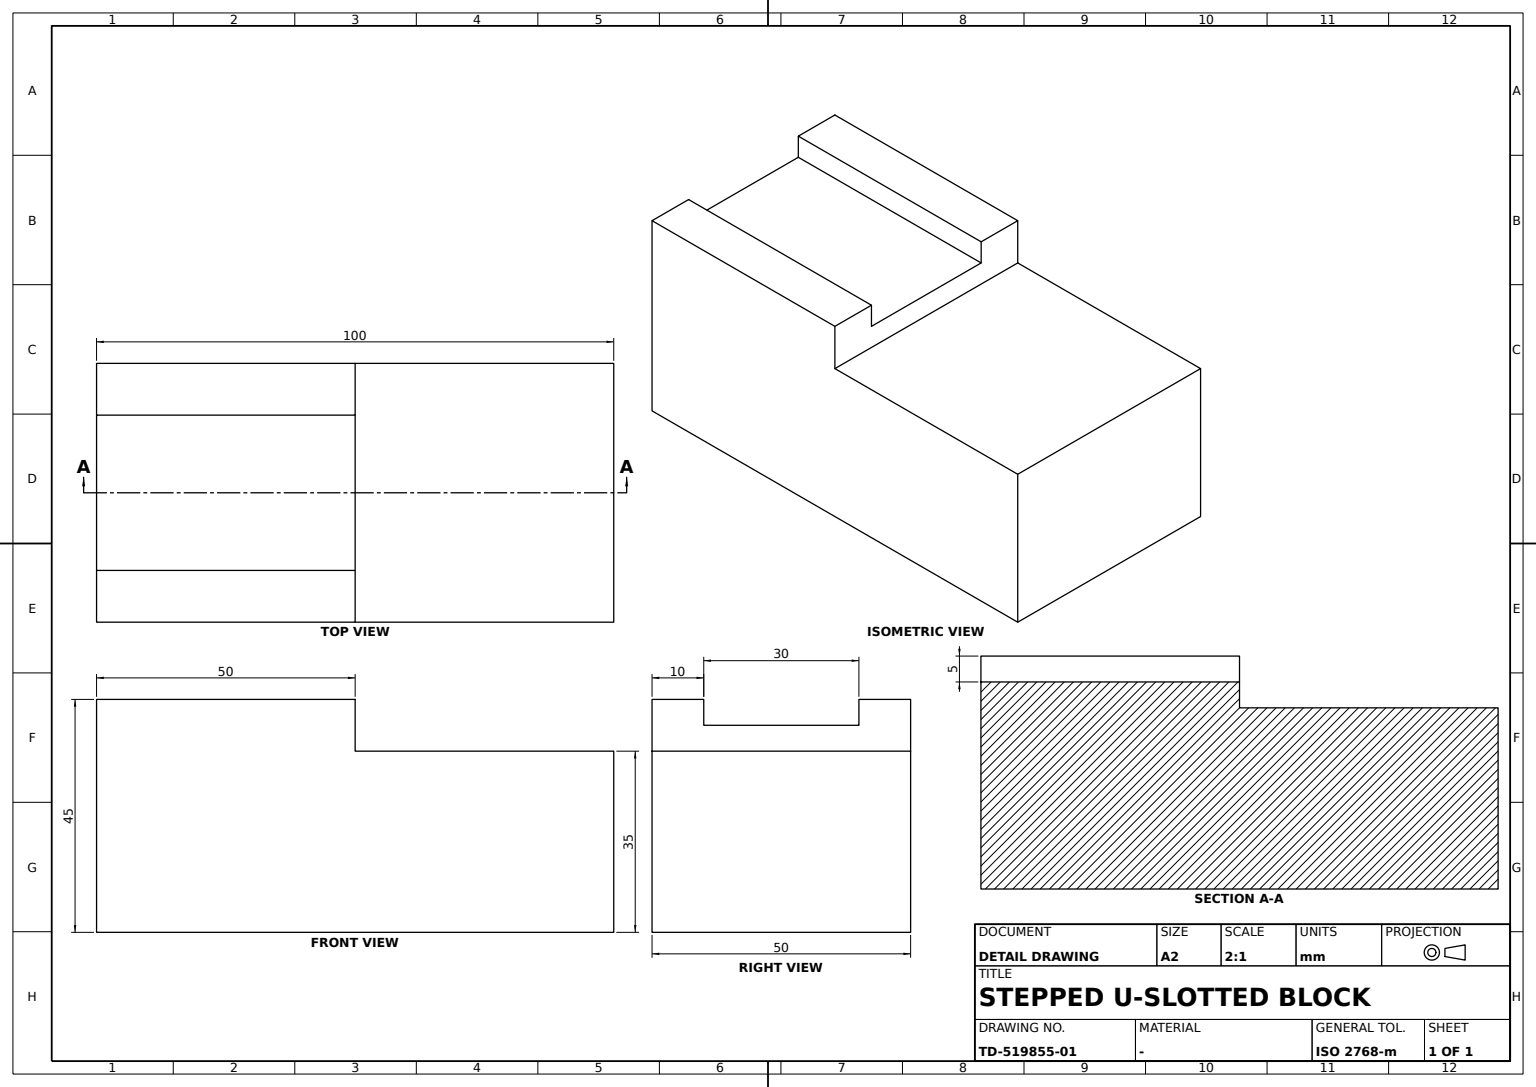
ISO-10303-21;
HEADER;
FILE_DESCRIPTION((''),'2;1');
FILE_NAME('','',(''),(''),'','','');
FILE_SCHEMA(('AUTOMOTIVE_DESIGN'));
ENDSEC;
DATA;
#1=APPLICATION_CONTEXT('');
#2=PRODUCT_CONTEXT('',#1,'mechanical');
#3=PRODUCT('','','',(#2));
#4=PRODUCT_DEFINITION_FORMATION('','',#3);
#5=PRODUCT_DEFINITION_CONTEXT('',#1,'design');
#6=PRODUCT_DEFINITION('','',#4,#5);
#7=PRODUCT_DEFINITION_SHAPE('','',#6);
#8=(LENGTH_UNIT()NAMED_UNIT(*)SI_UNIT(.MILLI.,.METRE.));
#9=(NAMED_UNIT(*)PLANE_ANGLE_UNIT()SI_UNIT($,.RADIAN.));
#10=(NAMED_UNIT(*)SI_UNIT($,.STERADIAN.)SOLID_ANGLE_UNIT());
#11=UNCERTAINTY_MEASURE_WITH_UNIT(LENGTH_MEASURE(1.E-05),#8,'distance_accuracy_value','');
#12=(GEOMETRIC_REPRESENTATION_CONTEXT(3)GLOBAL_UNCERTAINTY_ASSIGNED_CONTEXT((#11))GLOBAL_UNIT_ASSIGNED_CONTEXT((#8,#9,#10))REPRESENTATION_CONTEXT('',''));
#13=CARTESIAN_POINT('',(0.,-40.,5.));
#14=VERTEX_POINT('',#13);
#15=CARTESIAN_POINT('',(-50.,-40.,5.));
#16=VERTEX_POINT('',#15);
#17=CARTESIAN_POINT('',(-25.,-40.,5.));
#18=DIRECTION('',(-1.,0.,0.));
#19=VECTOR('',#18,1000.);
#20=LINE('',#17,#19);
#21=EDGE_CURVE('',#14,#16,#20,.T.);
#22=ORIENTED_EDGE('',*,*,#21,.F.);
#23=CARTESIAN_POINT('',(0.,-10.,5.));
#24=VERTEX_POINT('',#23);
#25=CARTESIAN_POINT('',(0.,-25.,5.));
#26=DIRECTION('',(0.,-1.,0.));
#27=VECTOR('',#26,1000.);
#28=LINE('',#25,#27);
#29=EDGE_CURVE('',#24,#14,#28,.T.);
#30=ORIENTED_EDGE('',*,*,#29,.F.);
#31=CARTESIAN_POINT('',(-50.,-10.,5.));
#32=VERTEX_POINT('',#31);
#33=CARTESIAN_POINT('',(-25.,-10.,5.));
#34=LINE('',#33,#19);
#35=EDGE_CURVE('',#24,#32,#34,.T.);
#36=ORIENTED_EDGE('',*,*,#35,.T.);
#37=CARTESIAN_POINT('',(-50.,-25.,5.));
#38=LINE('',#37,#27);
#39=EDGE_CURVE('',#32,#16,#38,.T.);
#40=ORIENTED_EDGE('',*,*,#39,.T.);
#41=EDGE_LOOP('',(#22,#30,#36,#40));
#42=FACE_OUTER_BOUND('',#41,.T.);
#43=DIRECTION('',(0.,0.,-1.));
#44=AXIS2_PLACEMENT_3D('',#23,#43,#26);
#45=PLANE('',#44);
#46=ADVANCED_FACE('',(#42),#45,.F.);
#47=ORIENTED_EDGE('',*,*,#35,.F.);
#48=CARTESIAN_POINT('',(0.,-10.,10.));
#49=VERTEX_POINT('',#48);
#50=CARTESIAN_POINT('',(0.,-10.,7.5));
#51=VECTOR('',#43,1000.);
#52=LINE('',#50,#51);
#53=EDGE_CURVE('',#49,#24,#52,.T.);
#54=ORIENTED_EDGE('',*,*,#53,.F.);
#55=CARTESIAN_POINT('',(-50.,-10.,10.));
#56=VERTEX_POINT('',#55);
#57=CARTESIAN_POINT('',(-25.,-10.,10.));
#58=LINE('',#57,#19);
#59=EDGE_CURVE('',#49,#56,#58,.T.);
#60=ORIENTED_EDGE('',*,*,#59,.T.);
#61=CARTESIAN_POINT('',(-50.,-10.,7.5));
#62=LINE('',#61,#51);
#63=EDGE_CURVE('',#56,#32,#62,.T.);
#64=ORIENTED_EDGE('',*,*,#63,.T.);
#65=EDGE_LOOP('',(#47,#54,#60,#64));
#66=FACE_OUTER_BOUND('',#65,.T.);
#67=DIRECTION('',(0.,1.,0.));
#68=AXIS2_PLACEMENT_3D('',#48,#67,#43);
#69=PLANE('',#68);
#70=ADVANCED_FACE('',(#66),#69,.F.);
#71=ORIENTED_EDGE('',*,*,#21,.T.);
#72=CARTESIAN_POINT('',(-50.,-40.,10.));
#73=VERTEX_POINT('',#72);
#74=CARTESIAN_POINT('',(-50.,-40.,7.5));
#75=DIRECTION('',(0.,0.,1.));
#76=VECTOR('',#75,1000.);
#77=LINE('',#74,#76);
#78=EDGE_CURVE('',#16,#73,#77,.T.);
#79=ORIENTED_EDGE('',*,*,#78,.T.);
#80=CARTESIAN_POINT('',(0.,-40.,10.));
#81=VERTEX_POINT('',#80);
#82=CARTESIAN_POINT('',(-25.,-40.,10.));
#83=LINE('',#82,#19);
#84=EDGE_CURVE('',#81,#73,#83,.T.);
#85=ORIENTED_EDGE('',*,*,#84,.F.);
#86=CARTESIAN_POINT('',(0.,-40.,7.5));
#87=LINE('',#86,#76);
#88=EDGE_CURVE('',#14,#81,#87,.T.);
#89=ORIENTED_EDGE('',*,*,#88,.F.);
#90=EDGE_LOOP('',(#71,#79,#85,#89));
#91=FACE_OUTER_BOUND('',#90,.T.);
#92=AXIS2_PLACEMENT_3D('',#13,#26,#75);
#93=PLANE('',#92);
#94=ADVANCED_FACE('',(#91),#93,.F.);
#95=CARTESIAN_POINT('',(50.,0.,0.));
#96=VERTEX_POINT('',#95);
#97=CARTESIAN_POINT('',(50.,-50.,0.));
#98=VERTEX_POINT('',#97);
#99=CARTESIAN_POINT('',(50.,-25.,0.));
#100=LINE('',#99,#27);
#101=EDGE_CURVE('',#96,#98,#100,.T.);
#102=ORIENTED_EDGE('',*,*,#101,.T.);
#103=CARTESIAN_POINT('',(50.,-50.,-35.));
#104=VERTEX_POINT('',#103);
#105=CARTESIAN_POINT('',(50.,-50.,-17.5));
#106=LINE('',#105,#51);
#107=EDGE_CURVE('',#98,#104,#106,.T.);
#108=ORIENTED_EDGE('',*,*,#107,.T.);
#109=CARTESIAN_POINT('',(50.,0.,-35.));
#110=VERTEX_POINT('',#109);
#111=CARTESIAN_POINT('',(50.,-25.,-35.));
#112=LINE('',#111,#27);
#113=EDGE_CURVE('',#110,#104,#112,.T.);
#114=ORIENTED_EDGE('',*,*,#113,.F.);
#115=CARTESIAN_POINT('',(50.,0.,-17.5));
#116=LINE('',#115,#51);
#117=EDGE_CURVE('',#96,#110,#116,.T.);
#118=ORIENTED_EDGE('',*,*,#117,.F.);
#119=EDGE_LOOP('',(#102,#108,#114,#118));
#120=FACE_OUTER_BOUND('',#119,.T.);
#121=AXIS2_PLACEMENT_3D('',#95,#18,#43);
#122=PLANE('',#121);
#123=ADVANCED_FACE('',(#120),#122,.F.);
#124=ORIENTED_EDGE('',*,*,#29,.T.);
#125=ORIENTED_EDGE('',*,*,#88,.T.);
#126=CARTESIAN_POINT('',(0.,-50.,10.));
#127=VERTEX_POINT('',#126);
#128=CARTESIAN_POINT('',(0.,-45.,10.));
#129=LINE('',#128,#27);
#130=EDGE_CURVE('',#81,#127,#129,.T.);
#131=ORIENTED_EDGE('',*,*,#130,.T.);
#132=CARTESIAN_POINT('',(0.,-50.,0.));
#133=VERTEX_POINT('',#132);
#134=CARTESIAN_POINT('',(0.,-50.,5.));
#135=LINE('',#134,#51);
#136=EDGE_CURVE('',#127,#133,#135,.T.);
#137=ORIENTED_EDGE('',*,*,#136,.T.);
#138=CARTESIAN_POINT('',(0.,0.,0.));
#139=VERTEX_POINT('',#138);
#140=CARTESIAN_POINT('',(0.,-25.,0.));
#141=VECTOR('',#67,1000.);
#142=LINE('',#140,#141);
#143=EDGE_CURVE('',#133,#139,#142,.T.);
#144=ORIENTED_EDGE('',*,*,#143,.T.);
#145=CARTESIAN_POINT('',(0.,0.,10.));
#146=VERTEX_POINT('',#145);
#147=CARTESIAN_POINT('',(0.,0.,5.));
#148=LINE('',#147,#76);
#149=EDGE_CURVE('',#139,#146,#148,.T.);
#150=ORIENTED_EDGE('',*,*,#149,.T.);
#151=CARTESIAN_POINT('',(0.,-5.,10.));
#152=LINE('',#151,#27);
#153=EDGE_CURVE('',#146,#49,#152,.T.);
#154=ORIENTED_EDGE('',*,*,#153,.T.);
#155=ORIENTED_EDGE('',*,*,#53,.T.);
#156=EDGE_LOOP('',(#124,#125,#131,#137,#144,#150,#154,#155));
#157=FACE_OUTER_BOUND('',#156,.T.);
#158=DIRECTION('',(1.,0.,0.));
#159=AXIS2_PLACEMENT_3D('',#138,#158,#67);
#160=PLANE('',#159);
#161=ADVANCED_FACE('',(#157),#160,.T.);
#162=ORIENTED_EDGE('',*,*,#63,.F.);
#163=CARTESIAN_POINT('',(-50.,0.,10.));
#164=VERTEX_POINT('',#163);
#165=CARTESIAN_POINT('',(-50.,-5.,10.));
#166=LINE('',#165,#27);
#167=EDGE_CURVE('',#164,#56,#166,.T.);
#168=ORIENTED_EDGE('',*,*,#167,.F.);
#169=CARTESIAN_POINT('',(-50.,0.,-35.));
#170=VERTEX_POINT('',#169);
#171=CARTESIAN_POINT('',(-50.,0.,-12.5));
#172=LINE('',#171,#76);
#173=EDGE_CURVE('',#170,#164,#172,.T.);
#174=ORIENTED_EDGE('',*,*,#173,.F.);
#175=CARTESIAN_POINT('',(-50.,-50.,-35.));
#176=VERTEX_POINT('',#175);
#177=CARTESIAN_POINT('',(-50.,-25.,-35.));
#178=LINE('',#177,#27);
#179=EDGE_CURVE('',#170,#176,#178,.T.);
#180=ORIENTED_EDGE('',*,*,#179,.T.);
#181=CARTESIAN_POINT('',(-50.,-50.,10.));
#182=VERTEX_POINT('',#181);
#183=CARTESIAN_POINT('',(-50.,-50.,-12.5));
#184=LINE('',#183,#76);
#185=EDGE_CURVE('',#176,#182,#184,.T.);
#186=ORIENTED_EDGE('',*,*,#185,.T.);
#187=CARTESIAN_POINT('',(-50.,-45.,10.));
#188=LINE('',#187,#27);
#189=EDGE_CURVE('',#73,#182,#188,.T.);
#190=ORIENTED_EDGE('',*,*,#189,.F.);
#191=ORIENTED_EDGE('',*,*,#78,.F.);
#192=ORIENTED_EDGE('',*,*,#39,.F.);
#193=EDGE_LOOP('',(#162,#168,#174,#180,#186,#190,#191,#192));
#194=FACE_OUTER_BOUND('',#193,.T.);
#195=AXIS2_PLACEMENT_3D('',#169,#158,#75);
#196=PLANE('',#195);
#197=ADVANCED_FACE('',(#194),#196,.F.);
#198=ORIENTED_EDGE('',*,*,#149,.F.);
#199=CARTESIAN_POINT('',(25.,0.,0.));
#200=VECTOR('',#158,1000.);
#201=LINE('',#199,#200);
#202=EDGE_CURVE('',#139,#96,#201,.T.);
#203=ORIENTED_EDGE('',*,*,#202,.T.);
#204=ORIENTED_EDGE('',*,*,#117,.T.);
#205=CARTESIAN_POINT('',(0.,0.,-35.));
#206=LINE('',#205,#19);
#207=EDGE_CURVE('',#110,#170,#206,.T.);
#208=ORIENTED_EDGE('',*,*,#207,.T.);
#209=ORIENTED_EDGE('',*,*,#173,.T.);
#210=CARTESIAN_POINT('',(-25.,0.,10.));
#211=LINE('',#210,#19);
#212=EDGE_CURVE('',#146,#164,#211,.T.);
#213=ORIENTED_EDGE('',*,*,#212,.F.);
#214=EDGE_LOOP('',(#198,#203,#204,#208,#209,#213));
#215=FACE_OUTER_BOUND('',#214,.T.);
#216=AXIS2_PLACEMENT_3D('',#138,#67,#18);
#217=PLANE('',#216);
#218=ADVANCED_FACE('',(#215),#217,.T.);
#219=ORIENTED_EDGE('',*,*,#202,.F.);
#220=ORIENTED_EDGE('',*,*,#143,.F.);
#221=CARTESIAN_POINT('',(25.,-50.,0.));
#222=LINE('',#221,#200);
#223=EDGE_CURVE('',#133,#98,#222,.T.);
#224=ORIENTED_EDGE('',*,*,#223,.T.);
#225=ORIENTED_EDGE('',*,*,#101,.F.);
#226=EDGE_LOOP('',(#219,#220,#224,#225));
#227=FACE_OUTER_BOUND('',#226,.T.);
#228=CARTESIAN_POINT('',(-50.,0.,0.));
#229=AXIS2_PLACEMENT_3D('',#228,#43,#158);
#230=PLANE('',#229);
#231=ADVANCED_FACE('',(#227),#230,.F.);
#232=ORIENTED_EDGE('',*,*,#130,.F.);
#233=ORIENTED_EDGE('',*,*,#84,.T.);
#234=ORIENTED_EDGE('',*,*,#189,.T.);
#235=CARTESIAN_POINT('',(-25.,-50.,10.));
#236=LINE('',#235,#19);
#237=EDGE_CURVE('',#127,#182,#236,.T.);
#238=ORIENTED_EDGE('',*,*,#237,.F.);
#239=EDGE_LOOP('',(#232,#233,#234,#238));
#240=FACE_OUTER_BOUND('',#239,.T.);
#241=AXIS2_PLACEMENT_3D('',#145,#43,#26);
#242=PLANE('',#241);
#243=ADVANCED_FACE('',(#240),#242,.F.);
#244=ORIENTED_EDGE('',*,*,#167,.T.);
#245=ORIENTED_EDGE('',*,*,#59,.F.);
#246=ORIENTED_EDGE('',*,*,#153,.F.);
#247=ORIENTED_EDGE('',*,*,#212,.T.);
#248=EDGE_LOOP('',(#244,#245,#246,#247));
#249=FACE_OUTER_BOUND('',#248,.T.);
#250=ADVANCED_FACE('',(#249),#242,.F.);
#251=CARTESIAN_POINT('',(0.,-50.,-35.));
#252=LINE('',#251,#19);
#253=EDGE_CURVE('',#104,#176,#252,.T.);
#254=ORIENTED_EDGE('',*,*,#253,.F.);
#255=ORIENTED_EDGE('',*,*,#107,.F.);
#256=ORIENTED_EDGE('',*,*,#223,.F.);
#257=ORIENTED_EDGE('',*,*,#136,.F.);
#258=ORIENTED_EDGE('',*,*,#237,.T.);
#259=ORIENTED_EDGE('',*,*,#185,.F.);
#260=EDGE_LOOP('',(#254,#255,#256,#257,#258,#259));
#261=FACE_OUTER_BOUND('',#260,.T.);
#262=AXIS2_PLACEMENT_3D('',#132,#67,#18);
#263=PLANE('',#262);
#264=ADVANCED_FACE('',(#261),#263,.F.);
#265=ORIENTED_EDGE('',*,*,#253,.T.);
#266=ORIENTED_EDGE('',*,*,#179,.F.);
#267=ORIENTED_EDGE('',*,*,#207,.F.);
#268=ORIENTED_EDGE('',*,*,#113,.T.);
#269=EDGE_LOOP('',(#265,#266,#267,#268));
#270=FACE_OUTER_BOUND('',#269,.T.);
#271=AXIS2_PLACEMENT_3D('',#109,#75,#18);
#272=PLANE('',#271);
#273=ADVANCED_FACE('',(#270),#272,.F.);
#274=CLOSED_SHELL('',(#46,#70,#94,#123,#161,#197,#218,#231,#243,#250,#264,#273));
#275=MANIFOLD_SOLID_BREP('',#274);
#276=ADVANCED_BREP_SHAPE_REPRESENTATION('',(#275),#12);
#277=SHAPE_DEFINITION_REPRESENTATION(#7,#276);
ENDSEC;
END-ISO-10303-21;
